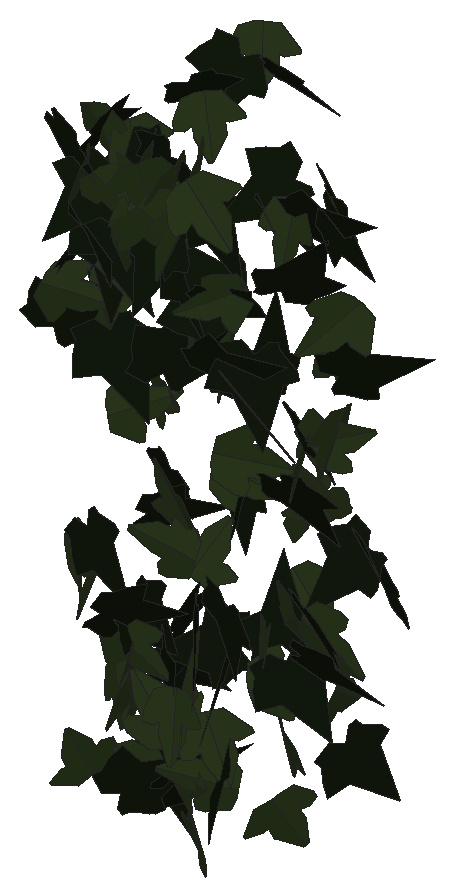
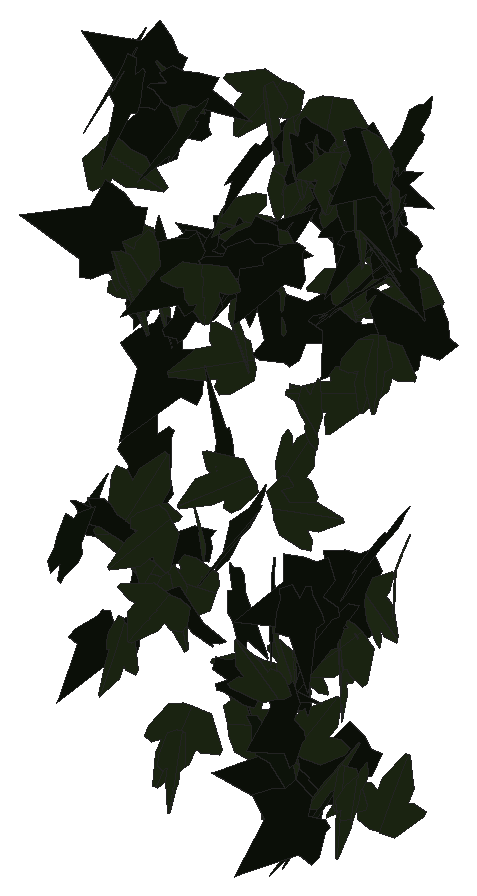
# SketchUp Ruby script. Lengths in inches.
U = 1.inch
M = Sketchup.active_model
def pt(a) = Geom::Point3d.new(a.map { |v| v * U })
def face(e, loops, mat)
  f = e.add_face(loops[0].map { |a| pt(a) })
  loops[1..].each { |l| e.add_face(l.map { |a| pt(a) }).erase! }
  f.material = f.back_material = mat if mat
  f
end
# faces: each face lists its corners as indices into pts; further lists are holes
def faces(e, pts, list, mat = nil) = list.each { |f| face(e, (f[0].is_a?(Array) ? f : [f]).map { |l| l.map { |i| pts[i] } }, mat) }
# xy, xz, yz: faces in a plane at the given z, y or x. An outline is a flat list of corners, or four numbers for a rectangle; further outlines are holes
def ring(l) = l.size == 4 ? [[l[0], l[1]], [l[2], l[1]], [l[2], l[3]], [l[0], l[3]]] : l.each_slice(2).to_a
def flat(e, list, mat, &to3) = list.each { |f| face(e, (f[0].is_a?(Array) ? f : [f]).map { |l| ring(l).map { |u, v| to3.(u, v) } }, mat) }
def xy(e, z, list, mat = nil) = flat(e, list, mat) { |x, y| [x, y, z] }
def xz(e, y, list, mat = nil) = flat(e, list, mat) { |x, z| [x, y, z] }
def yz(e, x, list, mat = nil) = flat(e, list, mat) { |y, z| [x, y, z] }
def lines(e, pts, list) = list.each { |a, b| e.add_line(pt(pts[a]), pt(pts[b])) }
# prism: a flat outline (further loops are holes) pulled along v
def prism(e, loops, v, mat = nil)
  f = face(e, loops, mat); d = Geom::Vector3d.new(v.map { |x| x * U })
  f.pushpull(f.normal.samedirection?(d) ? d.length : -d.length)
end
def box(e, o, s, mat = nil) = prism(e, [[o, [o[0] + s[0], o[1], o[2]], [o[0] + s[0], o[1] + s[1], o[2]], [o[0], o[1] + s[1], o[2]]]], [0, 0, s[2]], mat)
def at(x, y, z, deg = 0) = Geom::Transformation.translation(pt([x, y, z])) * Geom::Transformation.rotation(ORIGIN, Z_AXIS, deg.degrees)
def axes(o, x, y, z) = Geom::Transformation.new([*x, 0, *y, 0, *z, 0, *pt(o).to_a, 1])
def part(name) = M.definitions.add(name)
# library, detail: a bought-in or finely detailed component or shape, given as its bounding box
def library(name, o, s) = part(name).tap { |d| box(d.entities, o, s) }
def detail(e, o, s) = box(e.add_group.entities, o, s)
def put(e, d, t, mat = nil) = e.add_instance(d, t).tap { |i| i.material = mat if mat }
def group(e, t, mat = nil) = e.add_group.tap { |g| g.transformation = t; g.material = mat if mat }.entities
root = M.entities
M.materials.add("efeu1").color = [18, 25, 13]
M.materials.add("efeu2").color = [43, 57, 29]
c1 = part("ivyleaf_10")
p = [[0,0.5,-0.03],[-0.0625,2.02,-0.43],[-0.19,2.01,-0.46],[-0.54,1.05,-0.29],[-0.52,0.625,-0.18],[-0.83,0.76,-0.28],
  [-1.16,0.64,-0.33],[-1.15,0.33,-0.24],[-0.77,-0.39,0.02],[-0.3,-0.51,0.16],[0.04,-0.48,0.23],[-0.02,2.01,-0.4375],
  [-0.06,2.01,-0.43],[0.04,-0.49,0.23],[0.67,-0.49,0.14],[1.38,0.36,-0.2],[1.375,0.51,-0.24],[0.81,0.65,-0.19],
  [0.62,0.59,-0.15],[0.6,1.09,-0.28],[0.5,1.23,-0.31]]
faces(c1.entities,p,[[0,1,2,3,4,5,6,7,8,9,10],[11,12,0,13,14,15,16,17,18,19,20]],"efeu2")
c2 = part("ivyleaf_9")
p = [[1.54,2.16,1.25],[1.36,2.04,1.19],[-0.21,0.99,0.68],[-0.71,1.11,0.82],[-0.85,0.86,0.67],[-0.8,0.17,0.21],
  [-0.9,-0.01,0.1],[-0.67,-0.16,-0.02],[-0.08,-0.08,-0.05],[-0.03,-0.6,-0.4],[0.65,-0.88,-0.66],[0.83,-0.6,-0.49],
  [1.29,-0.42,-0.43],[1.8125,-0.07,-0.26],[1.21,0.44,0.15]]
faces(c2.entities,p,[[0,1,2,3,4,5,6,7,8,9,10,11,12,13,14]],"efeu1")
put(root,c1,axes([549.5,135.79,186.75],[-0.07427,0.82558,-0.12962],[0.01405,-0.12888,-0.82891],[-0.83558,-0.07555,-0.00242]))
put(root,c1,axes([549.89,134.43,199.7],[-0.72208,0.23643,0.34734],[-0.3233,0.12846,-0.75955],[-0.26836,-0.79091,-0.01954]))
put(root,c2,axes([550.21,134.92,204.68],[-0.49623,0.65289,-0.17433],[-0.00106,-0.21704,-0.80981],[-0.67576,-0.4791,0.12929]))
put(root,c1,axes([549.92,135.65,186.55],[0.1785,-0.81261,-0.54024],[-0.05083,0.54071,-0.83012],[0.97448,0.17706,0.05566]))
put(root,c2,axes([549.31,133.18,199.37],[-0.23075,-0.05903,0.8526],[0.83614,-0.19839,0.21256],[0.1769,0.86071,0.10747]))
put(root,c2,axes([549.73,138.9,204.96],[0.54697,0.62526,0.04511],[0.03068,0.03309,-0.83074],[-0.62614,0.54783,-0.0013]))
put(root,c2,axes([550.16,137.37,192.95],[0.44814,0.09059,-0.71612],[-0.70525,-0.12461,-0.45711],[-0.15377,0.83554,0.00947]))
put(root,c1,axes([549.89,134.24,199.46],[-0.68035,-0.43358,-0.179],[0.15106,0.09603,-0.80676],[0.44408,-0.69691,0.0002]))
put(root,c2,axes([549.48,133.05,206.11],[0.70496,-0.49975,-0.12423],[-0.08359,0.09677,-0.8636],[0.50813,0.70926,0.03029]))
put(root,c1,axes([550.08,133.77,184.7],[-0.42359,-0.63347,-0.44419],[-0.25101,-0.36649,0.76203],[-0.73183,0.49236,-0.00427]))
put(root,c1,axes([549.99,134.97,204.43],[0.30792,-0.75855,-0.17561],[0.00188,0.18957,-0.81555],[0.77862,0.29953,0.07142]))
put(root,c2,axes([550.23,133.25,202.57],[-0.36389,0.6912,-0.30489],[0.14581,-0.26779,-0.78112],[-0.74125,-0.392,-0.00398]))
put(root,c2,axes([549.99,134.12,205.52],[0.21336,0.53469,0.60036],[0.19373,0.56864,-0.57529],[-0.78025,0.2874,0.02132]))
put(root,c1,axes([550.12,133.43,204.85],[0.36006,-0.77432,-0.22314],[-0.04774,0.22348,-0.85251],[0.80441,0.35985,0.04929]))
put(root,c1,axes([549.81,134.46,205.91],[-0.72478,0.22806,-0.39044],[0.36759,-0.13238,-0.75968],[-0.26331,-0.81254,0.01418]))
put(root,c1,axes([549.63,132.78,200.93],[-0.32206,-0.20641,-0.80724],[0.72037,0.36593,-0.38097],[0.41871,-0.78832,0.03453]))
put(root,c1,axes([549.95,141.875,205.33],[0.73697,0.42686,0.03072],[0.01507,0.03524,-0.85136],[-0.4277,0.73677,0.02292]))
put(root,c2,axes([549.84,137.57,186.38],[0.69765,0.41356,0.2375],[0.20293,0.12341,-0.81101],[-0.43158,0.72656,0.00257]))
put(root,c1,axes([550.5,132.6,191.79],[-0.08994,0.37181,-0.81824],[-0.29845,0.76331,0.37965],[0.84776,0.30816,0.04685]))
put(root,c2,axes([550.78,134,203.15],[-0.42182,0.57027,0.48504],[-0.34071,0.34951,-0.70722],[-0.66663,-0.53948,0.05454]))
put(root,c2,axes([550.21,140.53,205.24],[-0.48185,-0.70197,0.06417],[-0.02598,-0.05998,-0.85134],[0.70441,-0.48239,0.01249]))
put(root,c1,axes([550.18,134.05,191.45],[0.30604,-0.68053,0.47277],[0.18468,-0.4353,-0.74613],[0.8078,0.35734,-0.00854]))
put(root,c2,axes([550.09,134.22,203.47],[0.23458,-0.46284,-0.67913],[-0.23603,0.63856,-0.51672],[0.78723,0.32938,0.04744]))
put(root,c2,axes([550.6,133.72,204.3],[-0.59801,-0.53068,0.26285],[-0.19704,-0.17398,-0.79953],[0.55847,-0.62964,-0.00062]))
put(root,c2,axes([550.0625,134.8,201.65],[0.31274,-0.76868,-0.21066],[0.14124,0.27616,-0.79802],[0.78441,0.25674,0.22768]))
put(root,c2,axes([550.25,134.58,201.68],[0.04744,-0.84082,0.1988],[0.0557,-0.19571,-0.84104],[0.8622,0.05891,0.0434]))
put(root,c2,axes([550.11,133.85,203.05],[0.29106,-0.77376,0.38072],[0.18108,-0.33802,-0.82542],[0.84313,0.33972,0.04585]))
put(root,c1,axes([551.46,133.43,202.83],[-0.31529,0.12301,0.8302],[-0.81806,0.15303,-0.33336],[-0.18745,-0.87477,0.05842]))
put(root,c1,axes([550.63,138.39,204.77],[0.68379,0.45294,0.15613],[0.12147,0.09929,-0.82005],[-0.46344,0.69432,0.01542]))
put(root,c2,axes([550.6,133.08,193.02],[0.47811,-0.6847,-0.38993],[-0.18718,0.34435,-0.83417],[0.76539,0.51192,0.03958]))
put(root,c1,axes([550.81,134.85,205.47],[0.30641,0.77243,0.13693],[0.02235,0.13835,-0.83045],[-0.78416,0.30577,0.02984]))
put(root,c2,axes([550.62,135.92,192.34],[0.49086,0.31504,0.62351],[0.51279,0.35502,-0.58307],[-0.47441,0.7097,0.01489]))
put(root,c2,axes([550.85,133.64,203.32],[-0.05095,-0.76734,-0.48789],[0.01109,0.48809,-0.76882],[0.90924,-0.04895,-0.01797]))
put(root,c1,axes([551.04,134.19,201.53],[0.6389,0.52676,-0.11076],[-0.07672,-0.08105,-0.82794],[-0.53279,0.64335,-0.01361]))
put(root,c2,axes([551.16,136.4375,188.48],[0.10531,0.39282,0.75518],[0.22527,0.72094,-0.40642],[-0.82088,0.24824,-0.01465]))
put(root,c1,axes([551.25,134.01,204.63],[0.74026,-0.37579,-0.26062],[-0.12998,0.30254,-0.80542],[0.43846,0.72414,0.20125]))
put(root,c1,axes([551.01,133.26,204.68],[-0.63843,-0.18733,-0.51249],[0.50008,0.11471,-0.6649],[0.21831,-0.8106,0.02435]))
put(root,c2,axes([551.84,134.46,205.11],[-0.80495,0.15235,0.20223],[-0.19579,0.05283,-0.8191],[-0.16055,-0.82828,-0.01504]))
put(root,c2,axes([550.83,141.24,204.89],[0.84244,-0.08607,0.1036],[0.11262,0.09021,-0.84085],[0.07388,0.84398,0.10044]))
put(root,c1,axes([551.54,133.79,189.2],[0.30296,-0.60334,-0.57966],[-0.20175,0.54562,-0.67335],[0.81199,0.36068,0.04898]))
put(root,c1,axes([551.04,137.64,190.0625],[0.75789,-0.00167,-0.39053],[0.38852,0.08979,0.75359],[0.03965,-0.84785,0.08058]))
put(root,c2,axes([551.15,133.45,199.57],[-0.2941,-0.5166,-0.75993],[0.4951,0.5831,-0.58799],[0.77411,-0.5692,0.08735]))
put(root,c2,axes([552.0625,136.3125,187.6875],[-0.4632,0.72519,0.08071],[-0.0483,0.06491,-0.86048],[-0.72807,-0.46568,0.00574]))
put(root,c2,axes([551.56,134.09,190.49],[0.25031,-0.40223,-0.72318],[-0.37689,0.61722,-0.47374],[0.73671,0.45242,0.00335]))
put(root,c1,axes([551.72,134.47,205.38],[0.25039,-0.78305,-0.18659],[0.00105,0.19573,-0.81998],[0.80497,0.24331,0.05911]))
put(root,c2,axes([551.23,135.42,184.8125],[0.58254,-0.7949,-0.16081],[-0.09514,0.12965,-0.98551],[0.80541,0.59026,-0.0001]))
put(root,c1,axes([551.86,134.33,184.97],[-0.34248,0.61,0.50448],[-0.00499,-0.55133,0.66326],[0.79157,0.26045,0.22245]))
put(root,c1,axes([551.64,134.12,203.5],[-0.29459,0.2219,0.81755],[0.30633,-0.7791,0.32184],[0.7898,0.38495,0.18011]))
put(root,c1,axes([551.52,133.54,189.58],[-0.64817,-0.09948,-0.60288],[0.59562,0.09329,-0.65576],[0.13637,-0.88028,-0.00137]))
put(root,c2,axes([552.47,134.4375,205.4375],[0.11108,0.16435,-0.82452],[-0.71123,-0.42512,-0.18055],[-0.44832,0.71515,0.08215]))
put(root,c2,axes([551.53,132.65,190.77],[0.55983,0.41629,0.59108],[0.48259,0.34146,-0.69757],[-0.53831,0.73905,-0.01065]))
put(root,c1,axes([551.61,133.37,197.25],[0.15155,0.04312,-0.8785],[0.66071,0.58285,0.14259],[0.58059,-0.67454,0.06705]))
put(root,c1,axes([551.5,135.05,197.11],[-0.18929,0.03868,0.8413],[0.80662,-0.23963,0.1925],[0.24218,0.82837,0.01641]))
put(root,c1,axes([552.39,134.46,186.46],[0.67108,0.56046,0.4478],[-0.36253,-0.26417,0.87394],[0.61904,-0.76229,0.02637]))
put(root,c1,axes([552.58,133.02,205.62],[-0.52869,-0.64272,-0.18805],[0.12955,0.13691,-0.83213],[0.65702,-0.54418,0.01275]))
put(root,c2,axes([552,132.95,184.875],[0.0656,0.02403,0.89967],[0.88257,0.17489,-0.06902],[-0.1762,0.88494,-0.01079]))
put(root,c1,axes([552.38,133.76,204.26],[0.33667,0.69136,0.43977],[0.16354,0.40918,-0.76847],[-0.80289,0.37325,0.02787]))
put(root,c2,axes([552.35,134.46,187.875],[-0.08296,0.16375,0.96435],[0.21921,-0.94008,0.17849],[0.95327,0.23042,0.04288]))
put(root,c1,axes([552.93,134.02,205.29],[0.09175,-0.86742,-0.15138],[-0.03846,0.14811,-0.87198],[0.87969,0.09695,-0.02234]))
put(root,c2,axes([552.88,133.72,203.25],[-0.73524,-0.30438,-0.28687],[0.27359,0.08885,-0.79547],[0.31637,-0.7842,0.02123]))
put(root,c2,axes([553.52,136.15,188.8125],[-0.6347,-0.02,0.59964],[-0.59955,-0.01162,-0.63499],[0.02252,-0.87308,-0.00529]))
put(root,c1,axes([553.57,133.73,193],[0.18279,0.12097,0.88791],[-0.84013,-0.29213,0.21275],[0.31176,-0.85817,0.05273]))
put(root,c1,axes([552.75,133.05,204.32],[-0.42194,-0.61089,-0.64139],[0.43578,0.47534,-0.73942],[0.77114,-0.60288,0.06691]))
put(root,c2,axes([552.8,133.88,198.78],[-0.34476,-0.24268,0.89029],[0.78375,0.42465,0.41926],[-0.48708,0.85507,0.04446]))
put(root,c1,axes([553.48,133.68,194.23],[-0.73094,0.32766,-0.41608],[-0.38691,0.15387,0.80086],[0.36164,0.82688,0.01585]))
put(root,c2,axes([552.8125,133.87,184.89],[0.04178,0.78909,-0.57645],[0.00413,0.57683,0.78991],[0.97722,-0.03617,0.02131]))
put(root,c2,axes([552.76,137.33,193.62],[0.18009,-0.80195,0.27016],[0.07251,-0.26057,-0.82182],[0.84312,0.1937,0.01298]))
put(root,c1,axes([553.32,134.01,203.82],[-0.03646,-0.78211,0.47728],[0.09444,-0.47832,-0.7766],[0.91136,0.01828,0.09957]))
put(root,c1,axes([553.69,134.25,199.74],[0.60572,-0.13981,0.59752],[-0.56818,0.18941,0.6203],[-0.23184,-0.82949,0.04093]))
put(root,c2,axes([553.23,134.34,202.09],[0.3095,-0.84912,-0.1149],[-0.03169,0.11074,-0.90373],[0.85627,0.31102,0.00809]))
put(root,c1,axes([553.49,133.93,188.33],[0.64805,-0.63701,0.0467],[-0.03246,0.03359,0.90871],[-0.63789,-0.64886,0.0012]))
put(root,c1,axes([553.5,133.33,188.14],[0.8843,-0.08577,0.18262],[0.1819,-0.01628,-0.88845],[0.08729,0.90281,0.00133]))
put(root,c1,axes([553.85,134.06,205.97],[0.33916,-0.78851,-0.23172],[-0.07065,0.22178,-0.85808],[0.81881,0.34575,0.02195]))
put(root,c2,axes([554.42,134.38,201.21],[-0.77462,-0.66786,-0.13671],[-0.09266,-0.10187,1.02265],[-0.67539,0.77997,0.01649]))
put(root,c1,axes([553.22,134.04,185.59],[0.07426,-0.04856,-0.90261],[0.68636,-0.58629,0.08801],[-0.58819,-0.69027,-0.01125]))
put(root,c2,axes([553.5,134.42,190.5],[-0.11533,-0.0041,-0.98294],[0.92078,-0.34684,-0.10659],[-0.34403,-0.92692,0.04423]))
put(root,c1,axes([553.86,135.53,199.49],[0.57281,-0.61177,0.40413],[0.28811,-0.28378,-0.83794],[0.67422,0.64101,0.01473]))
put(root,c1,axes([553.6875,135.73,194.85],[0.23018,0.28887,0.79062],[0.47476,0.63227,-0.36924],[-0.69507,0.52753,0.00961]))
put(root,c2,axes([554.47,134.2,201.65],[0.46413,0.58606,-0.43426],[-0.28689,-0.32656,-0.74734],[-0.67062,0.5453,0.01917]))
put(root,c2,axes([554.03,134.3,204.57],[0.38189,-0.74963,-0.42336],[-0.21216,0.36692,-0.84106],[0.83437,0.4364,-0.02009]))
put(root,c1,axes([554.97,133.79,185.78],[0.12435,0.08332,0.96406],[-0.80476,-0.53082,0.14968],[0.53732,-0.81431,0.00107]))
put(root,c1,axes([554.36,133.49,183.49],[-0.7117,0.50311,0.24217],[0.18494,-0.15779,0.87131],[0.52684,0.73503,0.02128]))
put(root,c1,axes([554.97,134.26,201.85],[0.17055,0.25103,-0.81469],[-0.70566,-0.42459,-0.27856],[-0.47831,0.71592,0.12047]))
put(root,c2,axes([554.75,134,186.73],[-0.54254,0.10059,-0.7366],[0.72691,-0.11945,-0.55171],[-0.1559,-0.90701,-0.00903]))
put(root,c1,axes([555.21,136.48,186.24],[-0.68007,0.42949,0.3523],[-0.28899,0.20207,-0.80419],[-0.47441,-0.73877,-0.01515]))
put(root,c1,axes([554.625,133.59,187.625],[0.70342,0.4508,0.34881],[0.28622,0.19977,-0.83538],[-0.49292,0.75932,0.01269]))
put(root,c2,axes([554.77,134.72,194.35],[-0.17948,0.75672,0.6815],[-0.00966,-0.69323,0.76721],[1.01832,0.12679,0.12739]))
put(root,c2,axes([555.02,134.14,190.1],[-0.58685,0.32547,-0.74128],[0.65434,-0.34843,-0.67101],[-0.47672,-0.87891,-0.00849]))
put(root,c1,axes([554.62,132.92,205.59],[0.57897,0.55131,0.53461],[0.39389,0.36155,-0.79943],[-0.65924,0.70021,-0.00814]))
put(root,c2,axes([555.51,135.82,189.89],[-0.88795,0.24223,0.00977],[0.00548,-0.01704,0.92027],[0.24236,0.88784,0.015]))
put(root,c1,axes([555.12,137.35,193.52],[-0.19967,-0.32645,-0.7891],[0.39444,0.6835,-0.38257],[0.7574,-0.44201,-0.00879]))
put(root,c1,axes([555.92,135.88,190.73],[-0.55731,0.18337,0.66664],[-0.64693,0.1638,-0.58589],[-0.24394,-0.85333,0.03079]))
put(root,c1,axes([555.17,137.125,191.09],[0.59786,0.39541,0.50622],[0.42127,0.28069,-0.71679],[-0.48491,0.73137,0.00141]))
put(root,c2,axes([555.72,135.02,198.92],[-0.29538,-0.50969,0.66162],[0.39569,0.53261,0.58696],[-0.73549,0.49124,0.05008]))
put(root,c2,axes([555.16,133.73,191.71],[0.25146,-0.74354,0.48384],[0.14082,-0.46307,-0.7848],[0.87585,0.28792,-0.01273]))
put(root,c1,axes([556.11,137.17,193.82],[-0.72287,-0.25905,-0.43576],[-0.40749,-0.15457,0.76785],[-0.30158,0.82978,0.007]))
put(root,c2,axes([555.05,133.2,199.74],[0.21918,-0.14525,0.87945],[0.84881,-0.24247,-0.25159],[0.27212,0.87332,0.07642]))
put(root,c1,axes([555.51,133.45,196.96],[0.10903,0.1087,0.91296],[0.57684,0.70781,-0.15317],[-0.71594,0.58685,0.01563]))
put(root,c2,axes([556.625,134.91,205.93],[-0.7893,-0.25026,0.31227],[-0.30289,-0.07768,-0.82786],[0.26153,-0.84526,-0.01637]))
put(root,c2,axes([555.8,135.0625,205.0625],[0.65686,-0.51269,-0.28318],[-0.14379,0.27133,-0.82475],[0.56777,0.66184,0.11875]))
put(root,c1,axes([556.79,133.39,190.57],[0.27824,-0.21537,0.86431],[-0.69131,0.5188,0.35182],[-0.56171,-0.74518,-0.00486]))
put(root,c2,axes([556.31,133.6,200.47],[-0.45498,-0.61852,-0.52069],[0.31595,0.41394,-0.7678],[0.74422,-0.55387,0.00764]))
put(root,c2,axes([555.93,133.22,199.4],[0.73751,-0.49471,0.29596],[0.24355,-0.16819,-0.88805],[0.5225,0.77667,-0.0038]))
put(root,c1,axes([556.72,134.2,185.47],[-0.47026,-0.68373,-0.44092],[0.25637,0.35879,-0.82981],[0.77212,-0.53556,0.00699]))
put(root,c1,axes([557.36,136.05,200.4],[0.70124,-0.45029,-0.44963],[-0.34974,0.28624,-0.83212],[0.53161,0.78229,0.04566]))
put(root,c1,axes([556.52,133.86,189.61],[0.24896,0.06479,-0.89605],[0.8439,0.30203,0.25631],[0.30812,-0.87958,0.022]))
put(root,c1,axes([557.4,136.13,188.76],[0.02161,-0.54033,-0.71714],[-0.00245,0.71731,-0.54053],[0.89791,0.01496,0.01578]))
put(root,c2,axes([557.68,136.95,193.07],[-0.87697,-0.16565,0.00713],[-0.00676,-0.00261,-0.89248],[0.16567,-0.87699,0.00131]))
put(root,c1,axes([557.25,134.04,205.38],[0.87882,-0.18659,0.06142],[0.06068,-0.00995,-0.89841],[0.18684,0.88091,0.00286]))
put(root,c2,axes([557.41,133.625,196.64],[0.96652,0.27053,-0.15593],[-0.15026,-0.04166,-1.00367],[-0.27372,0.97813,0.00038]))
put(root,c2,axes([557.69,135.29,205.88],[0.66879,-0.11344,-0.57789],[-0.55606,0.16634,-0.67618],[0.19395,0.86808,0.05405]))
put(root,c2,axes([557.61,133.55,190.79],[-0.05118,-0.60134,-0.66443],[0.1838,0.64432,-0.5973],[0.87709,-0.17011,0.0864]))
put(root,c2,axes([557.63,133.34,203.37],[0.80587,0.55117,0.07252],[-0.08654,-0.00178,0.97519],[0.54915,-0.80913,0.04725]))
put(root,c2,axes([558.29,137.62,191.58],[0.41025,-0.78844,0.32455],[-0.12451,0.30091,0.88839],[-0.84349,-0.42789,0.02672]))
put(root,c1,axes([558.1875,133.54,198.28],[0.49972,-0.75757,0.09475],[0.05943,-0.0743,-0.90749],[0.76115,0.50316,0.00865]))
put(root,c1,axes([557.67,134.82,191.47],[-0.45257,0.17463,-0.92439],[0.85816,-0.34364,-0.48507],[-0.38543,-0.97017,0.00542]))
put(root,c2,axes([558.04,133.88,198.42],[0.71191,-0.36236,-0.50729],[0.45602,-0.22236,0.79879],[-0.42508,-0.84541,0.00734]))
put(root,c2,axes([557.8,134.16,205.32],[0.27974,-0.26078,0.81831],[0.78603,-0.26908,-0.35445],[0.34611,0.82187,0.1436]))
put(root,c2,axes([558.77,132.96,193.18],[0.82508,0.0021,-0.56346],[-0.5614,0.08855,-0.82173],[0.04821,0.99519,0.07431]))
put(root,c1,axes([559.2,134.34,202.63],[0.49904,0.40218,-0.6925],[-0.61783,-0.32577,-0.63443],[-0.50949,0.78897,0.09104]))
put(root,c2,axes([558.66,134.15,205.8],[0.62133,-0.43191,-0.50206],[-0.35964,0.35803,-0.75308],[0.55612,0.71409,0.07392]))
put(root,c2,axes([558.31,133.46,191.28],[0.80184,-0.15088,0.38349],[0.384,-0.03099,-0.81509],[0.1496,0.88829,0.03671]))
put(root,c2,axes([558.83,134.78,187.98],[0.07537,-0.38418,-0.80255],[-0.1627,0.7859,-0.39148],[0.87477,0.17927,-0.00367]))
put(root,c1,axes([559.27,133.73,199.375],[0.16572,-0.91126,0.2276],[0.062,-0.22,-0.92597],[0.93721,0.17569,0.02101]))
put(root,c1,axes([558.77,133.49,198.52],[-0.3352,-0.23085,0.82015],[0.67139,0.47106,0.40699],[-0.52458,0.75041,-0.00318]))
put(root,c2,axes([558.66,134.75,200.24],[0.34967,0.00643,0.87388],[0.86408,0.13813,-0.34677],[-0.13061,0.93105,0.04542]))
